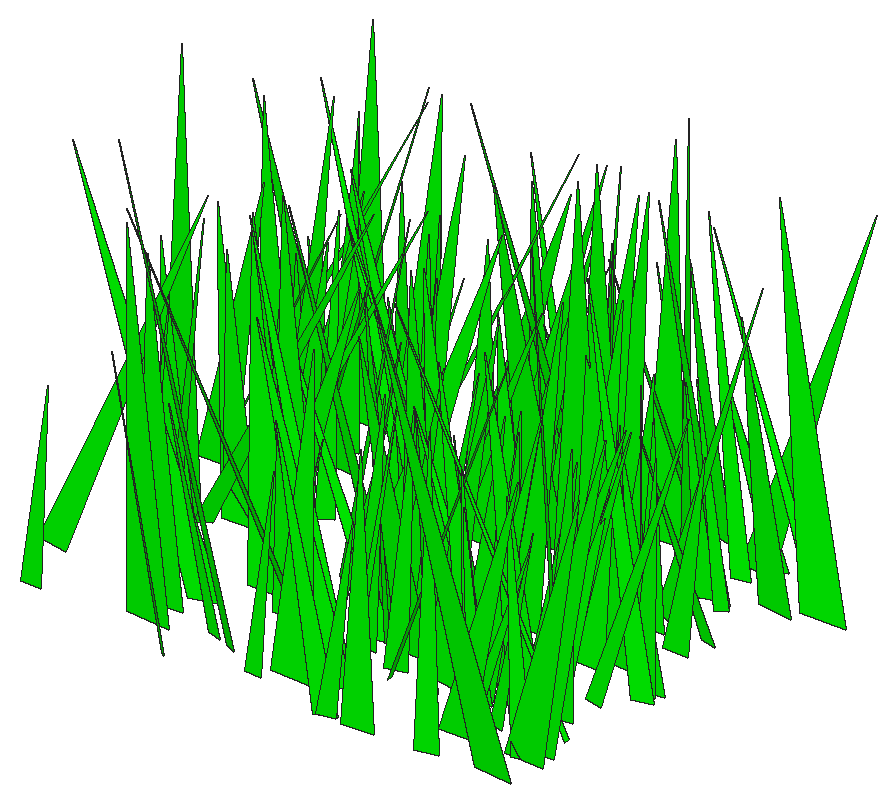
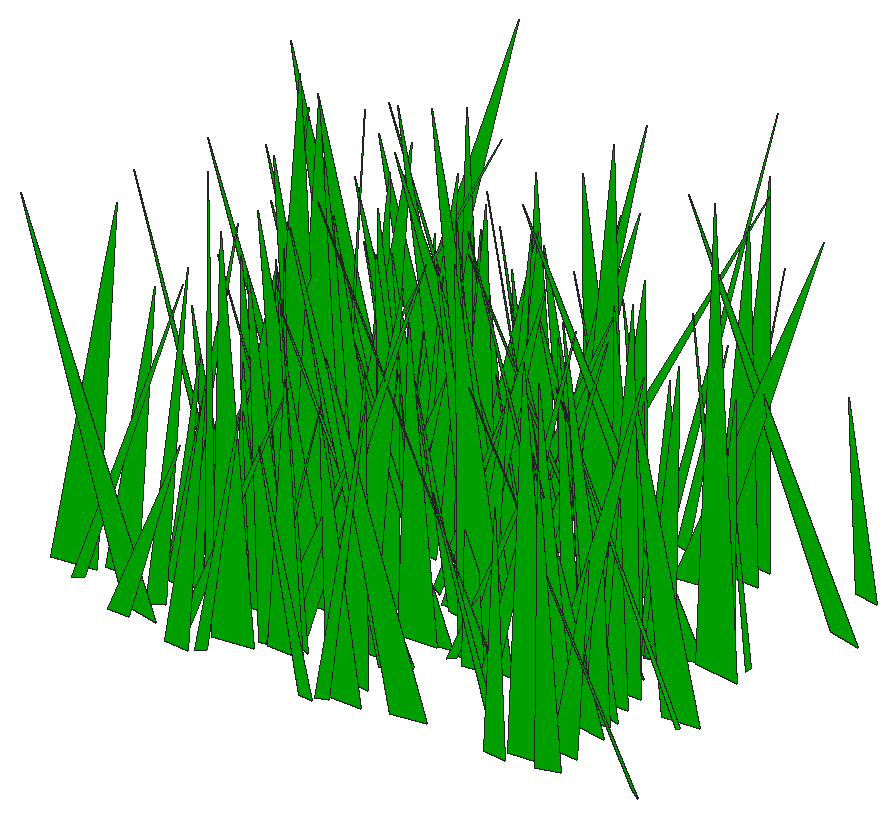
# SketchUp Ruby script. Lengths in inches.
U = 1.inch
M = Sketchup.active_model
def pt(a) = Geom::Point3d.new(a.map { |v| v * U })
def face(e, loops, mat)
  f = e.add_face(loops[0].map { |a| pt(a) })
  loops[1..].each { |l| e.add_face(l.map { |a| pt(a) }).erase! }
  f.material = f.back_material = mat if mat
  f
end
# faces: each face lists its corners as indices into pts; further lists are holes
def faces(e, pts, list, mat = nil) = list.each { |f| face(e, (f[0].is_a?(Array) ? f : [f]).map { |l| l.map { |i| pts[i] } }, mat) }
# xy, xz, yz: faces in a plane at the given z, y or x. An outline is a flat list of corners, or four numbers for a rectangle; further outlines are holes
def ring(l) = l.size == 4 ? [[l[0], l[1]], [l[2], l[1]], [l[2], l[3]], [l[0], l[3]]] : l.each_slice(2).to_a
def flat(e, list, mat, &to3) = list.each { |f| face(e, (f[0].is_a?(Array) ? f : [f]).map { |l| ring(l).map { |u, v| to3.(u, v) } }, mat) }
def xy(e, z, list, mat = nil) = flat(e, list, mat) { |x, y| [x, y, z] }
def xz(e, y, list, mat = nil) = flat(e, list, mat) { |x, z| [x, y, z] }
def yz(e, x, list, mat = nil) = flat(e, list, mat) { |y, z| [x, y, z] }
def lines(e, pts, list) = list.each { |a, b| e.add_line(pt(pts[a]), pt(pts[b])) }
# prism: a flat outline (further loops are holes) pulled along v
def prism(e, loops, v, mat = nil)
  f = face(e, loops, mat); d = Geom::Vector3d.new(v.map { |x| x * U })
  f.pushpull(f.normal.samedirection?(d) ? d.length : -d.length)
end
def box(e, o, s, mat = nil) = prism(e, [[o, [o[0] + s[0], o[1], o[2]], [o[0] + s[0], o[1] + s[1], o[2]], [o[0], o[1] + s[1], o[2]]]], [0, 0, s[2]], mat)
def at(x, y, z, deg = 0) = Geom::Transformation.translation(pt([x, y, z])) * Geom::Transformation.rotation(ORIGIN, Z_AXIS, deg.degrees)
def axes(o, x, y, z) = Geom::Transformation.new([*x, 0, *y, 0, *z, 0, *pt(o).to_a, 1])
def part(name) = M.definitions.add(name)
# library, detail: a bought-in or finely detailed component or shape, given as its bounding box
def library(name, o, s) = part(name).tap { |d| box(d.entities, o, s) }
def detail(e, o, s) = box(e.add_group.entities, o, s)
def put(e, d, t, mat = nil) = e.add_instance(d, t).tap { |i| i.material = mat if mat }
def group(e, t, mat = nil) = e.add_group.tap { |g| g.transformation = t; g.material = mat if mat }.entities
root = M.entities
M.materials.add("[0065_Lime]").color = [0, 255, 0]
c1 = part("fur_instance\#9")
p = [[0.8125,0,1.79],[0.67,-0.02,1.48],[0,-0.11,0],[0,0.11,0]]
faces(c1.entities,p,[[0,1,2,3]])
put(root,c1,axes([108.63,19.34,1.48],[2.01758,0.4866,0.68769],[-3.49798,0.29654,-0.24089],[-0.68596,-0.08096,3.25107]),"[0065_Lime]")
put(root,c1,axes([108.67,24.51,1.48],[4.02995,-0.02811,1.22036],[0.35063,0.60062,-0.30247],[-1.4724,0.06609,3.26808]),"[0065_Lime]")
put(root,c1,axes([109.59,24.6875,1.48],[-2.13126,0.68575,1.17407],[-5.06141,-0.30855,-0.04016],[0.53076,-0.18874,4.33146]),"[0065_Lime]")
put(root,c1,axes([109.25,25.22,1.48],[5.27062,0.92734,3.1835],[-7.30081,0.81135,0.07783],[-2.35982,-0.43894,6.86953]),"[0065_Lime]")
put(root,c1,axes([108.28,28,1.48],[2.86012,-0.78922,0.70468],[5.68059,0.40097,-0.20671],[-0.16421,0.12475,5.12265]),"[0065_Lime]")
put(root,c1,axes([109.68,31.41,1.48],[-0.15102,-0.58534,0.1046],[4.16198,-0.02025,0.17925],[-0.21568,0.01916,3.38582]),"[0065_Lime]")
put(root,c1,axes([106.76,31.93,1.48],[7.32872,0.24015,0.08147],[-1.70459,1.02935,-0.22089],[-0.15916,0.03397,6.11724]),"[0065_Lime]")
put(root,c1,axes([109.49,32.39,1.48],[4.40549,-0.45639,2.09936],[3.71321,0.6697,-0.27704],[-1.84992,0.25738,4.44345]),"[0065_Lime]")
put(root,c1,axes([111.3,29.8,1.48],[-5.25137,-0.72724,1.01769],[5.26664,-0.74577,0.12315],[0.78312,0.13875,5.9961]),"[0065_Lime]")
put(root,c1,axes([110.06,29.46,1.48],[-0.7372,0.51936,1.26984],[-4.00435,-0.10917,-0.04194],[0.2506,-0.21664,3.06532]),"[0065_Lime]")
put(root,c1,axes([107.66,21.51,1.48],[6.7982,0.72444,0.23139],[-5.15748,0.95588,-0.02584],[-0.24586,-0.02059,6.93997]),"[0065_Lime]")
put(root,c1,axes([110.17,32.23,1.48],[-2.6226,1.00884,1.99234],[-7.48634,-0.40298,0.31731],[1.22409,-0.30311,6.20918]),"[0065_Lime]")
put(root,c1,axes([110.27,28.42,1.48],[-0.73571,-0.56275,0.68],[4.07523,-0.11133,-0.17018],[0.36092,0.10996,3.30774]),"[0065_Lime]")
put(root,c1,axes([108.13,28.3125,1.48],[6.20146,0.01374,0.29438],[-0.12343,0.87063,0.35909],[-0.35398,-0.06293,5.03218]),"[0065_Lime]")
put(root,c1,axes([109.89,24.09,1.48],[5.74407,0.29229,1.78391],[-2.25124,0.85529,0.10022],[-2.01708,-0.1222,4.96822]),"[0065_Lime]")
put(root,c1,axes([110.91,25.65,1.48],[3.72719,-0.50219,2.78782],[4.44047,0.60571,-0.27179],[-2.19109,0.37329,4.19145]),"[0065_Lime]")
put(root,c1,axes([110.75,27.6875,1.48],[-3.59681,0.86773,2.5202],[-6.77868,-0.53808,-0.19295],[1.33512,-0.39428,5.80975]),"[0065_Lime]")
put(root,c1,axes([113,21.64,1.48],[-6.99231,0.6663,0.53071],[-4.77212,-0.98301,-0.24472],[0.37029,-0.08652,6.86775]),"[0065_Lime]")
put(root,c1,axes([109.91,30,1.48],[2.82424,0.70846,0.1928],[-5.03033,0.39821,-0.27815],[-0.41422,-0.0055,4.69242]),"[0065_Lime]")
put(root,c1,axes([111.07,27.04,1.48],[1.16724,-0.70043,1.99344],[5.47562,0.2042,0.28285],[-0.93284,0.32217,4.15463]),"[0065_Lime]")
put(root,c1,axes([110.22,28.97,1.48],[5.40336,0.71175,1.69235],[-5.18229,0.79735,-0.2893],[-1.76882,-0.16184,6.01738]),"[0065_Lime]")
put(root,c1,axes([110.98,25.71,1.48],[1.05286,-0.76879,0.86109],[5.5426,0.16015,0.30731],[-0.57722,0.13553,4.52149]),"[0065_Lime]")
put(root,c1,axes([110.51,30.71,1.48],[3.60819,-0.78274,1.30441],[5.68647,0.52947,0.23922],[-1.1249,0.16583,5.39326]),"[0065_Lime]")
put(root,c1,axes([111.15,32.69,1.48],[-2.91426,-0.4897,1.54004],[3.73538,-0.44985,-0.11639],[1.33286,0.19001,3.69342]),"[0065_Lime]")
put(root,c1,axes([111.28,27.88,1.48],[2.17546,-0.65229,1.3075],[4.90065,0.30529,-0.29133],[-0.34057,0.22641,4.15979]),"[0065_Lime]")
put(root,c1,axes([112.16,20.71,1.48],[0.76189,-0.93665,1.74244],[6.98366,0.12326,0.19978],[-0.49926,0.29475,5.45364]),"[0065_Lime]")
put(root,c1,axes([112.4,19.82,1.48],[-3.14117,-0.93645,2.13884],[7.08142,-0.46703,0.02918],[1.08662,0.3365,5.99275]),"[0065_Lime]")
put(root,c1,axes([113.95,29.48,1.48],[-7.52353,0.25642,1.27269],[-1.80631,-1.07973,0.22449],[1.58594,-0.01334,6.29317]),"[0065_Lime]")
put(root,c1,axes([110.86,28.97,1.48],[8.68715,0.06479,1.33231],[-0.4,1.24156,-0.29763],[-1.65391,0.04006,7.06992]),"[0065_Lime]")
put(root,c1,axes([112.67,27.35,1.48],[5.40993,-0.35328,1.74258],[2.53261,0.81449,0.33098],[-2.12045,0.07148,4.84118]),"[0065_Lime]")
put(root,c1,axes([113.93,18.58,1.48],[-5.42349,-0.112,1.20908],[0.88853,-0.78757,0.19251],[1.4336,0.06443,4.45476]),"[0065_Lime]")
put(root,c1,axes([115.1875,20.01,1.48],[-9.0122,-0.28904,1.64617],[2.17807,-1.29309,0.28156],[1.89281,0.11178,7.51389]),"[0065_Lime]")
put(root,c1,axes([110.14,25.09,1.48],[8.00053,-0.33266,0.00856],[2.36563,1.12356,0.23417],[-0.09178,-0.03837,6.78263]),"[0065_Lime]")
put(root,c1,axes([112.32,31.3,1.48],[4.14379,-0.08843,0.54905],[0.62886,0.58991,0.0436],[-0.67544,0.0067,3.40898]),"[0065_Lime]")
put(root,c1,axes([114.1,23.14,1.48],[-2.16113,0.98291,0.03037],[-6.99025,-0.30367,0.21026],[0.25799,0.00571,5.95141]),"[0065_Lime]")
put(root,c1,axes([114.89,26.78,1.48],[-5.72751,-0.42516,0.83048],[3.02785,-0.81666,-0.1932],[1.01447,0.03709,5.2654]),"[0065_Lime]")
put(root,c1,axes([113.25,24.14,1.48],[2.64816,0.66717,2.07874],[-5.31558,0.39015,0.28441],[-0.90483,-0.33942,4.413]),"[0065_Lime]")
put(root,c1,axes([114.41,20.28,1.48],[-3.73431,-0.30458,0.7595],[2.19906,-0.5382,-0.07853],[0.85693,0.05384,3.51128]),"[0065_Lime]")
put(root,c1,axes([115.51,29.1,1.48],[-5.44204,0.14229,0.34665],[-0.99659,-0.76672,0.19446],[0.46245,0.02218,4.49841]),"[0065_Lime]")
put(root,c1,axes([110.84,26.62,1.48],[7.4321,0.31518,0.1034],[-2.24456,1.04435,0.07328],[-0.09565,-0.01728,6.31426]),"[0065_Lime]")
put(root,c1,axes([112.43,25.66,1.48],[4.20385,-0.63472,0.28642],[4.52778,0.59098,-0.08524],[-0.16301,0.04626,5.01848]),"[0065_Lime]")
put(root,c1,axes([117.81,20.63,1.48],[-8.11436,-0.33888,0.0616],[2.41282,-1.13939,0.25027],[-0.01511,0.04447,6.88113]),"[0065_Lime]")
put(root,c1,axes([114.47,28.92,1.48],[0.99322,1.2442,0.14911],[-8.85171,0.1403,-0.21689],[-0.28546,-0.02141,7.24422]),"[0065_Lime]")
put(root,c1,axes([114.68,29.22,1.48],[4.40952,-0.3902,1.75757],[2.97735,0.6732,0.06583],[-1.87486,0.15136,4.2382]),"[0065_Lime]")
put(root,c1,axes([117.08,26.83,1.48],[-5.77869,0.66661,0.7874],[-4.78734,-0.81833,-0.03131],[0.72356,-0.09052,6.08142]),"[0065_Lime]")
put(root,c1,axes([115.64,22.46,1.48],[2.23319,-1.06597,2.34203],[8.01924,0.35391,0.33836],[-1.23665,0.37001,6.42347]),"[0065_Lime]")
put(root,c1,axes([115.95,27.34,1.48],[-1.92642,-0.60241,1.31022],[4.5675,-0.27061,0.2741],[0.3336,0.22644,3.81319]),"[0065_Lime]")
put(root,c1,axes([114.84,26.2,1.48],[4.5332,-0.00086,1.00689],[-0.03962,0.65987,0.13682],[-1.23724,-0.02427,3.68483]),"[0065_Lime]")
put(root,c1,axes([115.75,27.78,1.48],[2.07017,0.50392,0.88749],[-3.6852,0.30564,-0.12777],[-0.68576,-0.12127,3.36575]),"[0065_Lime]")
put(root,c1,axes([114.3125,32.53,1.48],[3.89962,-0.7769,0.22289],[5.53466,0.54632,-0.25971],[0.10337,0.05731,5.4972]),"[0065_Lime]")
put(root,c1,axes([116.87,33.16,1.48],[-5.8235,0.21409,1.52227],[-1.63959,-0.85504,-0.12039],[1.77074,-0.08761,4.89487]),"[0065_Lime]")
put(root,c1,axes([115.49,27.73,1.48],[-4.26882,-0.5974,3.42126],[5.32235,-0.71065,0.23576],[2.72731,0.45178,4.89493]),"[0065_Lime]")
put(root,c1,axes([118.32,22.98,1.48],[-5.43651,0.34578,0.12997],[-2.45281,-0.76386,0.2148],[0.25435,0.02457,4.84929]),"[0065_Lime]")
put(root,c1,axes([115.17,24.97,1.48],[7.34613,0.20855,1.68148],[-1.57912,1.06947,0.11995],[-1.99556,-0.07858,6.09498]),"[0065_Lime]")
put(root,c1,axes([116.78,31.93,1.48],[-2.91777,-0.69369,2.02044],[5.42122,-0.4359,0.16502],[1.07273,0.31609,4.66156]),"[0065_Lime]")
put(root,c1,axes([118.22,26.38,1.48],[-5.35983,-0.19894,0.6505],[1.4784,-0.75738,0.2982],[0.67691,0.07896,4.49941]),"[0065_Lime]")
put(root,c1,axes([113.66,29.31,1.48],[8.70341,0.22956,0.33053],[-1.61805,1.22371,-0.28875],[-0.46461,0.03855,7.19732]),"[0065_Lime]")
put(root,c1,axes([118.51,20.68,1.48],[-7.81581,0.41713,1.50993],[-3.05642,-1.12412,-0.06168],[1.70769,-0.10281,6.80031]),"[0065_Lime]")
put(root,c1,axes([116.6,19.25,1.48],[2.8111,0.40797,0.85431],[-2.93288,0.41522,-0.25903],[-0.96468,-0.07354,3.27697]),"[0065_Lime]")
put(root,c1,axes([116.3,32.92,1.48],[1.9292,-0.74087,0.18561],[5.2748,0.27176,0.07393],[-0.16383,0.02572,4.56613]),"[0065_Lime]")
put(root,c1,axes([116.85,28.96,1.48],[0.49858,-0.82835,1.55366],[6.19661,0.0654,-0.1473],[0.02872,0.26957,4.8099]),"[0065_Lime]")
put(root,c1,axes([118.8,20.14,1.48],[-4.79635,0.69722,0.38612],[-4.96852,-0.67616,0.07664],[0.39779,-0.03873,5.61285]),"[0065_Lime]")
put(root,c1,axes([117.12,26.3,1.48],[-4.5605,-0.69268,2.55914],[5.3562,-0.71979,-0.21303],[2.34724,0.29667,5.45833]),"[0065_Lime]")
put(root,c1,axes([116.67,20.18,1.48],[4.32396,0.25892,0.85307],[-1.78942,0.62521,-0.35766],[-1.13718,0.00072,3.80644]),"[0065_Lime]")
put(root,c1,axes([116.98,27.14,1.48],[3.41785,0.30596,0.84269],[-2.24555,0.49588,-0.00691],[-0.87846,-0.07718,3.29633]),"[0065_Lime]")
put(root,c1,axes([117.99,23.61,1.48],[-5.08829,-0.5219,1.65789],[3.79749,-0.76029,-0.30858],[1.87836,0.1233,5.11492]),"[0065_Lime]")
put(root,c1,axes([119.77,30.52,1.48],[-7.6797,-0.46999,0.94744],[3.35532,-1.09059,-0.13365],[1.13392,0.04397,6.81221]),"[0065_Lime]")
put(root,c1,axes([116.01,28.8125,1.48],[5.13192,-0.30999,0.28977],[2.19119,0.72267,0.22948],[-0.43851,-0.01675,4.53792]),"[0065_Lime]")
put(root,c1,axes([118.37,29.97,1.48],[-1.88113,-1.01337,0.52374],[7.23907,-0.265,0.02169],[0.13662,0.0885,6.06231]),"[0065_Lime]")
put(root,c1,axes([116.88,22.49,1.48],[4.45608,-0.12078,0.82072],[0.90395,0.64062,-0.08836],[-0.96937,0.0422,3.69039]),"[0065_Lime]")
put(root,c1,axes([117.52,25.41,1.48],[4.68351,0.54174,1.88588],[-4.12843,0.70441,0.00311],[-1.78741,-0.20749,4.93432]),"[0065_Lime]")
put(root,c1,axes([117.5625,19.75,1.48],[-0.02768,0.9052,1.39266],[-6.65784,-0.01531,0.24587],[0.32011,-0.24013,5.23419]),"[0065_Lime]")
put(root,c1,axes([116.73,25.79,1.48],[7.22743,-0.74699,1.9113],[5.46979,1.05233,0.09637],[-1.96525,0.18175,7.29724]),"[0065_Lime]")
put(root,c1,axes([117.28,33.4,1.48],[3.86501,0.34038,0.98422],[-2.56934,0.55454,0.24946],[-0.85445,-0.12787,3.70186]),"[0065_Lime]")
put(root,c1,axes([118.44,22.9,1.48],[-3.77961,-0.16215,1.32762],[1.38708,-0.56599,0.29638],[1.43926,0.11966,3.20078]),"[0065_Lime]")
put(root,c1,axes([118.71,19.23,1.48],[-4.47618,-0.1095,1.17696],[0.71099,-0.66089,-0.27134],[1.48169,-0.01369,3.68578]),"[0065_Lime]")
put(root,c1,axes([115.95,30.29,1.48],[6.54917,0.07841,0.32208],[-0.55644,0.92195,-0.03483],[-0.39816,0.00128,5.34637]),"[0065_Lime]")
put(root,c1,axes([116.375,30.67,1.48],[7.28139,-0.49262,0.98807],[3.53088,1.03552,0.08385],[-1.13961,0.06084,6.57297]),"[0065_Lime]")
put(root,c1,axes([117.92,22.43,1.48],[2.17965,0.59255,1.68503],[-4.66819,0.3094,0.34946],[-0.53088,-0.28777,3.84537]),"[0065_Lime]")
put(root,c1,axes([118.96,27.89,1.48],[-0.86773,0.74098,0.13154],[-5.27205,-0.12094,-0.18251],[-0.19526,-0.02752,4.34313]),"[0065_Lime]")
put(root,c1,axes([118.63,24.17,1.48],[0.46551,-0.90236,2.32628],[7.01799,0.08294,0.1489],[-0.40646,0.39862,5.2351]),"[0065_Lime]")
put(root,c1,axes([116.68,24.51,1.48],[4.18103,1.06681,0.03694],[-7.58759,0.58689,0.2648],[0.26327,-0.02765,7.04501]),"[0065_Lime]")
put(root,c1,axes([119.43,22.85,1.48],[-2.61004,-0.81259,0.65958],[5.83212,-0.36899,0.03694],[0.29184,0.1065,5.16063]),"[0065_Lime]")
put(root,c1,axes([118.39,30.24,1.48],[1.78625,0.51411,0.35829],[-3.65246,0.25613,-0.26713],[-0.48945,-0.03507,3.30098]),"[0065_Lime]")
put(root,c1,axes([117.14,30.35,1.48],[5.24049,-0.65853,0.42025],[4.6723,0.73989,0.30117],[-0.63206,0.00944,5.71064]),"[0065_Lime]")
put(root,c1,axes([119.61,18.69,1.48],[-4.20901,0.45454,1.23315],[-3.45435,-0.60177,-0.36839],[0.91064,-0.18181,4.30219]),"[0065_Lime]")
put(root,c1,axes([119.52,24.33,1.48],[-2.26505,0.93766,0.94387],[-6.76635,-0.3209,-0.06129],[0.30065,-0.15784,5.73166]),"[0065_Lime]")
put(root,c1,axes([120.08,30.93,1.48],[-2.52826,-0.49216,0.31266],[3.52097,-0.35037,0.35738],[-0.13384,0.07984,3.49545]),"[0065_Lime]")
put(root,c1,axes([119.3,31.74,1.48],[-0.04385,0.78764,0.91071],[-5.71474,-0.00276,-0.10223],[-0.1194,-0.15742,4.55838]),"[0065_Lime]")
put(root,c1,axes([120.13,31.64,1.48],[-4.85316,-0.20533,0.89754],[1.39735,-0.69916,-0.36051],[1.18329,-0.0165,4.10688]),"[0065_Lime]")
put(root,c1,axes([118.51,21.34,1.48],[5.25846,-0.07386,1.32002],[0.65572,0.76976,-0.28501],[-1.57476,0.07388,4.28916]),"[0065_Lime]")
put(root,c1,axes([119.84,24.99,1.48],[-2.56677,-0.62145,0.83199],[4.509,-0.36811,-0.00955],[0.52378,0.12346,4.15935]),"[0065_Lime]")
put(root,c1,axes([118.63,23.1,1.48],[4.00505,0.56332,1.10137],[-4.11056,0.58012,-0.05254],[-1.00389,-0.12799,4.60908]),"[0065_Lime]")
put(root,c1,axes([118.99,31.32,1.48],[6.7838,0.27385,2.17549],[-2.15206,1.01625,0.15353],[-2.5139,-0.13099,5.73917]),"[0065_Lime]")
put(root,c1,axes([119.53,21.93,1.48],[-3.67702,0.38925,2.31958],[-3.37802,-0.5937,-0.20452],[2.09629,-0.27395,3.73911]),"[0065_Lime]")
put(root,c1,axes([119.64,18.66,1.48],[2.955,-0.40256,0.77103],[2.92788,0.42761,0.05671],[-0.73027,0.08548,3.34731]),"[0065_Lime]")
put(root,c1,axes([119.66,31.63,1.48],[4.36943,-0.73131,1.85646],[5.52394,0.64156,-0.13353],[-1.33446,0.26119,5.52587]),"[0065_Lime]")
put(root,c1,axes([121.23,33.08,1.48],[-4.76139,0.18584,1.07242],[-1.29921,-0.69412,0.21395],[1.34138,-0.01265,4.0139]),"[0065_Lime]")
put(root,c1,axes([122.16,22.93,1.48],[-4.6571,0.2953,0.32039],[-2.09222,-0.65674,0.16153],[0.44068,0.00276,4.15284]),"[0065_Lime]")
put(root,c1,axes([121.04,21.63,1.48],[-4.48812,-0.31021,1.55731],[2.35628,-0.6758,-0.01782],[1.7283,0.11578,4.0684]),"[0065_Lime]")
put(root,c1,axes([122.57,32.07,1.48],[-5.25427,-0.28365,0.38675],[2.02577,-0.74095,0.00003],[0.44383,0.02397,4.57844]),"[0065_Lime]")
put(root,c1,axes([120.79,18.625,1.48],[-2.38896,0.6318,1.86959],[-4.91643,-0.37254,0.06207],[1.15226,-0.27966,4.14102]),"[0065_Lime]")
put(root,c1,axes([120.79,32.21,1.48],[-4.65972,0.78909,2.81037],[-6.16042,-0.73293,0.13767],[2.34979,-0.35671,5.93398]),"[0065_Lime]")
put(root,c1,axes([120.57,29.18,1.48],[1.71315,1.11657,0.64408],[-7.98467,0.24116,0.04265],[-0.11538,-0.11032,6.61187]),"[0065_Lime]")
put(root,c1,axes([121.48,22.95,1.48],[-4.05284,-0.2626,1.23942],[1.89909,-0.60566,-0.1913],[1.48584,0.05782,3.62519]),"[0065_Lime]")
put(root,c1,axes([120.61,23.97,1.48],[3.79933,-0.50435,0.70627],[3.57355,0.54627,0.35246],[-0.93064,0.03863,4.23675]),"[0065_Lime]")
put(root,c1,axes([121.18,29.17,1.48],[-6.14944,-0.05317,2.4014],[0.28567,-0.95836,-0.227],[2.96265,-0.01795,5.00635]),"[0065_Lime]")
put(root,c1,axes([120.8,25.98,1.48],[3.76281,0.75812,1.23524],[-5.49859,0.54913,-0.21089],[-1.08628,-0.1535,5.34629]),"[0065_Lime]")
put(root,c1,axes([121.23,30.3125,1.48],[-0.48255,0.56963,0.50751],[-4.07354,-0.07686,0.32808],[0.47855,-0.07985,3.30446]),"[0065_Lime]")
put(root,c1,axes([121.91,33.32,1.48],[-3.51076,-0.55716,1.04942],[4.01413,-0.51574,-0.29018],[1.12822,0.10122,4.29801]),"[0065_Lime]")
put(root,c1,axes([122.43,21.86,1.48],[3.86392,-0.57069,2.6347],[4.5363,0.64709,0.29499],[-2.5314,0.28849,4.55023]),"[0065_Lime]")
put(root,c1,axes([120.77,22.19,1.48],[-4.20865,-0.6665,3.47224],[5.61438,-0.72828,-0.18182],[3.03295,0.42327,5.1548]),"[0065_Lime]")
put(root,c1,axes([119.69,21.43,1.48],[7.34774,0.0286,0.81409],[-0.19175,1.04197,-0.08173],[-1.00316,0.01035,5.97848]),"[0065_Lime]")
put(root,c1,axes([121.85,27.12,1.48],[-0.30731,-1.23261,1.92172],[9.07945,-0.05278,-0.17373],[0.30374,0.33059,7.13748]),"[0065_Lime]")
put(root,c1,axes([121.79,23.67,1.48],[0.19962,0.73864,0.70661],[-5.32498,0.02365,0.16711],[0.17513,-0.123,4.27557]),"[0065_Lime]")
put(root,c1,axes([122,31.71,1.48],[7.73171,0.32863,3.03136],[-2.77485,1.1859,0.37479],[-3.41438,-0.21962,6.55978]),"[0065_Lime]")
put(root,c1,axes([122.9375,24.74,1.48],[7.1747,0.18582,3.08678],[-1.59109,1.13337,0.16066],[-3.69027,-0.12739,5.93212]),"[0065_Lime]")
put(root,c1,axes([125.74,21.73,1.48],[-7.98055,-0.01854,0.1858],[0.13164,-1.12187,-0.01014],[0.2286,-0.00122,6.49236]),"[0065_Lime]")
put(root,c1,axes([123.04,21.03,1.48],[-3.13149,0.49759,0.94361],[-3.57627,-0.46114,0.29575],[1.04666,-0.0869,3.83372]),"[0065_Lime]")
put(root,c1,axes([122.78,26.99,1.48],[2.37801,-1.19167,2.70133],[9.03994,0.36754,0.16775],[-1.10861,0.44084,7.16233]),"[0065_Lime]")
put(root,c1,axes([122.25,25.16,1.48],[0.85511,0.53131,1.02433],[-3.98071,0.1052,0.37022],[0.19091,-0.18623,3.13145]),"[0065_Lime]")
put(root,c1,axes([122.44,22.98,1.48],[1.00306,-0.77407,0.58062],[5.55427,0.1384,-0.16604],[0.07466,0.10379,4.55151]),"[0065_Lime]")
put(root,c1,axes([123.27,20.86,1.48],[2.70431,-0.36694,1.56978],[2.87563,0.43455,0.126],[-1.50805,0.17061,3.05527]),"[0065_Lime]")
put(root,c1,axes([123.15,28.26,1.48],[-4.25472,-0.01329,1.53683],[0.2788,-0.65075,0.32215],[1.87107,0.06675,3.44668]),"[0065_Lime]")
put(root,c1,axes([124.16,30.6,1.48],[-6.75478,-0.42885,1.59292],[3.09441,-0.98501,-0.20422],[1.89051,0.07998,6.02576]),"[0065_Lime]")
put(root,c1,axes([124.32,32.87,1.48],[-2.81495,0.42113,0.33363],[-3.02475,-0.39103,-0.34618],[-0.03245,-0.08293,3.32652]),"[0065_Lime]")
put(root,c1,axes([123.1,18.79,1.48],[4.98847,-0.42793,2.11929],[3.35946,0.76524,-0.05424],[-2.1856,0.19951,4.75377]),"[0065_Lime]")
put(root,c1,axes([123.82,31.84,1.48],[5.77713,-0.25156,2.9691],[2.33346,0.93499,-0.34953],[-3.32923,0.2188,4.90722]),"[0065_Lime]")
put(root,c1,axes([122.26,22.21,1.48],[3.74025,0.66031,0.78598],[-4.75732,0.53271,-0.01783],[-0.61913,-0.10429,4.88527]),"[0065_Lime]")
put(root,c1,axes([124.0625,22.0625,1.48],[-4.22539,0.72925,1.47296],[-5.40561,-0.60947,-0.14884],[0.9959,-0.21407,5.44159]),"[0065_Lime]")
put(root,c1,axes([123.71,30.42,1.48],[-2.70177,0.38467,1.31095],[-3.06109,-0.39473,-0.29295],[0.84921,-0.19902,3.11482]),"[0065_Lime]")
put(root,c1,axes([123.59,28.11,1.48],[-0.70086,0.6016,0.1029],[-4.27965,-0.09909,0.12706],[0.17465,-0.01398,3.52656]),"[0065_Lime]")
put(root,c1,axes([125.34,18.94,1.48],[-5.92621,-0.8915,1.02842],[6.44013,-0.83581,0.27598],[0.61184,0.16262,7.05637]),"[0065_Lime]")
put(root,c1,axes([123.32,25.38,1.48],[1.79781,1.04626,0.50874],[-7.4659,0.25517,-0.12868],[-0.30105,-0.08018,6.22918]),"[0065_Lime]")
put(root,c1,axes([124.49,30.14,1.48],[-3.75212,0.25378,1.33685],[-2.09565,-0.55198,-0.38044],[1.25344,-0.16319,3.36574]),"[0065_Lime]")
put(root,c1,axes([124.03,25.93,1.48],[-0.93977,-0.60802,1.54565],[4.69028,-0.15334,-0.13442],[0.57875,0.25538,3.59918]),"[0065_Lime]")
put(root,c1,axes([123.08,20.76,1.48],[3.85212,-0.23877,0.4641],[1.72301,0.54564,-0.05552],[-0.49416,0.04121,3.42423]),"[0065_Lime]")
put(root,c1,axes([122.62,24.58,1.48],[4.90285,-0.44596,0.35012],[3.17232,0.69141,0.11824],[-0.44043,0.01566,4.74919]),"[0065_Lime]")
put(root,c1,axes([125.35,28.47,1.48],[-3.21861,-0.34704,0.08672],[2.45927,-0.45202,-0.22196],[0.25057,-0.02133,3.2925]),"[0065_Lime]")
put(root,c1,axes([123.71,21.11,1.48],[3.29166,0.32848,0.77039],[-2.38092,0.47688,-0.08253],[-0.83229,-0.06509,3.28293]),"[0065_Lime]")
put(root,c1,axes([123.1,20.09,1.48],[3.33914,-0.67712,0.61972],[4.87708,0.46656,-0.30489],[-0.12236,0.11807,4.75898]),"[0065_Lime]")
put(root,c1,axes([126.45,31.98,1.48],[-6.77662,0.18175,0.77301],[-1.29379,-0.96147,0.07083],[0.94988,-0.0129,5.61126]),"[0065_Lime]")
put(root,c1,axes([126.01,24.75,1.48],[-7.14709,0.40172,1.79043],[-2.93452,-1.04652,0.11765],[2.09921,-0.09522,6.26027]),"[0065_Lime]")
put(root,c1,axes([123.35,28.95,1.48],[6.85417,0.35972,1.09961],[-2.64317,0.97675,0.19399],[-1.18088,-0.09835,5.94827]),"[0065_Lime]")
put(root,c1,axes([125.39,20.14,1.48],[-3.91682,0.37599,1.56215],[-2.93139,-0.58913,-0.11169],[1.50157,-0.16935,3.85683]),"[0065_Lime]")
put(root,c1,axes([124.67,22.55,1.48],[2.28714,-0.76981,0.54722],[5.49769,0.32682,0.20299],[-0.49072,0.07356,4.82468]),"[0065_Lime]")
put(root,c1,axes([123.94,25.63,1.48],[4.62257,0.20307,0.55545],[-1.44233,0.65649,-0.10048],[-0.68876,-0.01189,3.93824]),"[0065_Lime]")
put(root,c1,axes([124.35,22.73,1.48],[1.29808,0.67338,0.16045],[-4.7817,0.17947,0.35665],[0.37217,-0.04277,4.02266]),"[0065_Lime]")
put(root,c1,axes([125.66,31.05,1.48],[-2.54744,-0.74332,0.81319],[5.34079,-0.36848,-0.21673],[0.67683,0.10996,4.77087]),"[0065_Lime]")
put(root,c1,axes([125.87,25.28,1.48],[-1.39958,0.59677,1.24816],[-4.51566,-0.18557,-0.37704],[0.01225,-0.22524,3.6177]),"[0065_Lime]")
put(root,c1,axes([123.96,23.38,1.48],[5.6082,-0.3952,0.64268],[2.78744,0.79583,0.30483],[-0.87433,0.00224,5.09416]),"[0065_Lime]")
put(root,c1,axes([124.96,27.5,1.48],[1.71707,-0.52451,0.89199],[3.88852,0.2367,-0.28867],[-0.12287,0.16104,3.32959]),"[0065_Lime]")
put(root,c1,axes([123.83,32.52,1.48],[5.8509,0.81772,0.40098],[-5.81307,0.82485,-0.24483],[-0.56192,-0.01877,6.70792]),"[0065_Lime]")
put(root,c1,axes([125.72,25.13,1.48],[2.21657,0.56591,0.95306],[-4.10562,0.33084,-0.26489],[-0.85795,-0.12111,3.72988]),"[0065_Lime]")
put(root,c1,axes([127.04,31.44,1.48],[-4.25532,0.98244,0.67701],[-6.9962,-0.60536,0.3414],[0.79253,-0.06895,6.64881]),"[0065_Lime]")
put(root,c1,axes([124.97,23.87,1.48],[5.65162,0.44757,0.63761],[-3.17761,0.80147,-0.21638],[-0.81387,-0.02123,5.27247]),"[0065_Lime]")
put(root,c1,axes([125.49,20.14,1.48],[2.20417,-0.84223,0.11304],[5.98401,0.30778,-0.36093],[0.3687,0.03981,5.18205]),"[0065_Lime]")
put(root,c1,axes([125.43,20.64,1.48],[4.27561,-0.82937,0.6931],[5.95619,0.60118,-0.20503],[-0.29406,0.11783,5.92474]),"[0065_Lime]")
